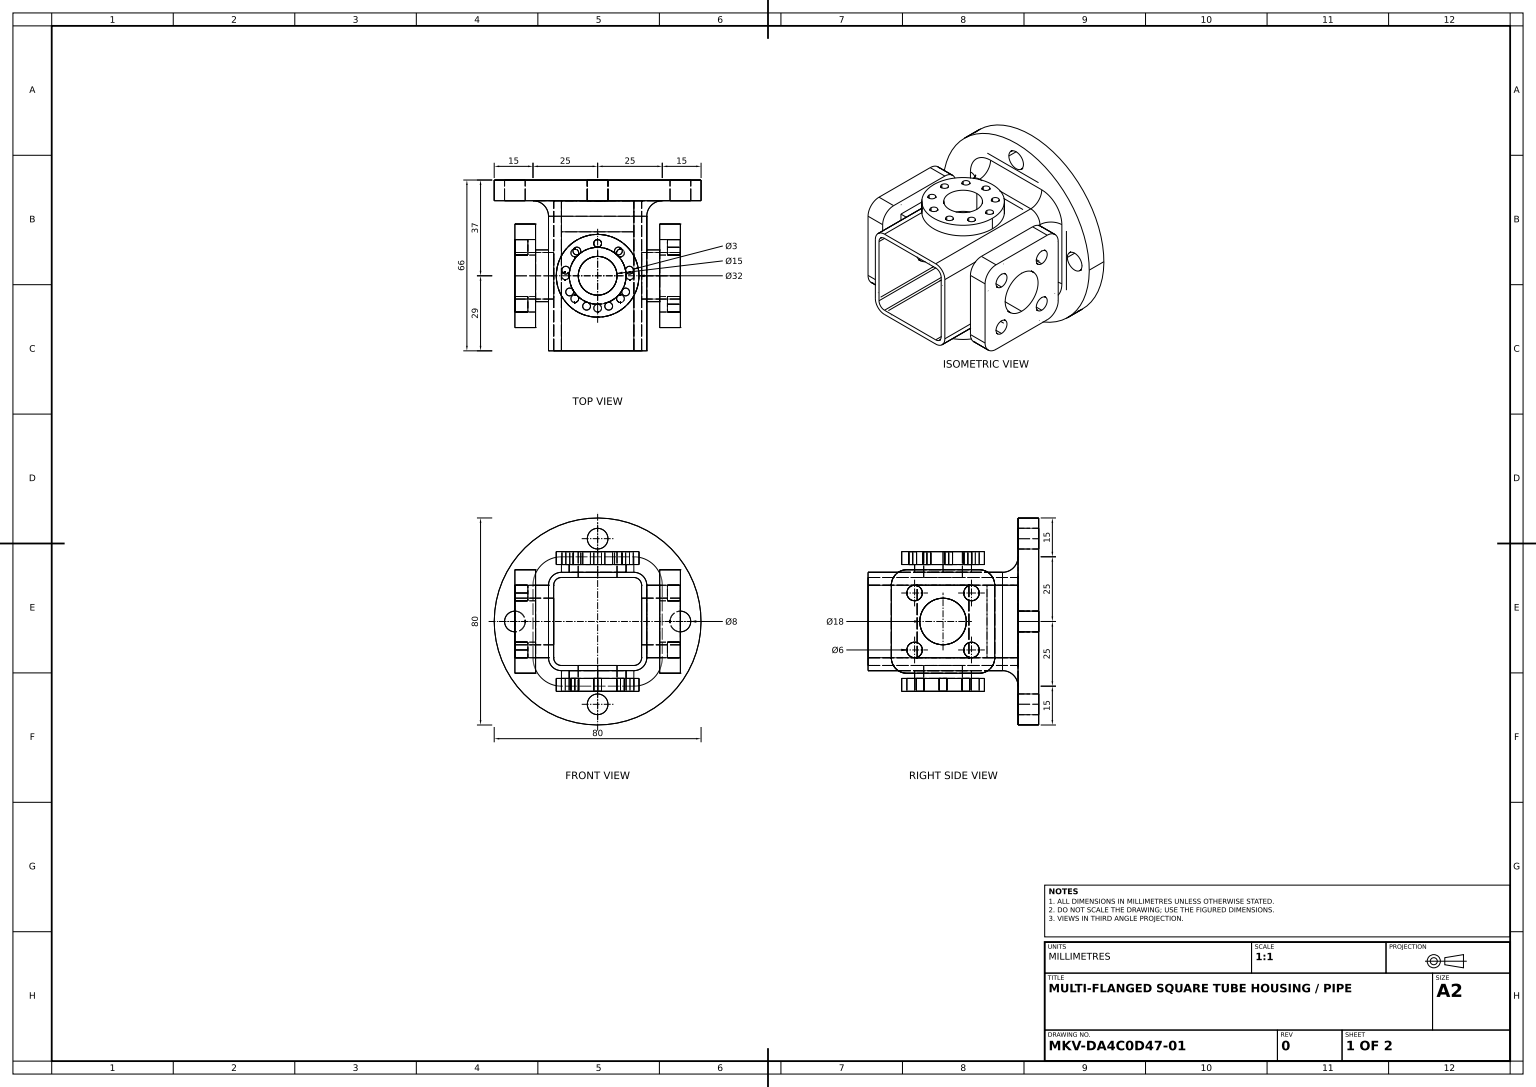
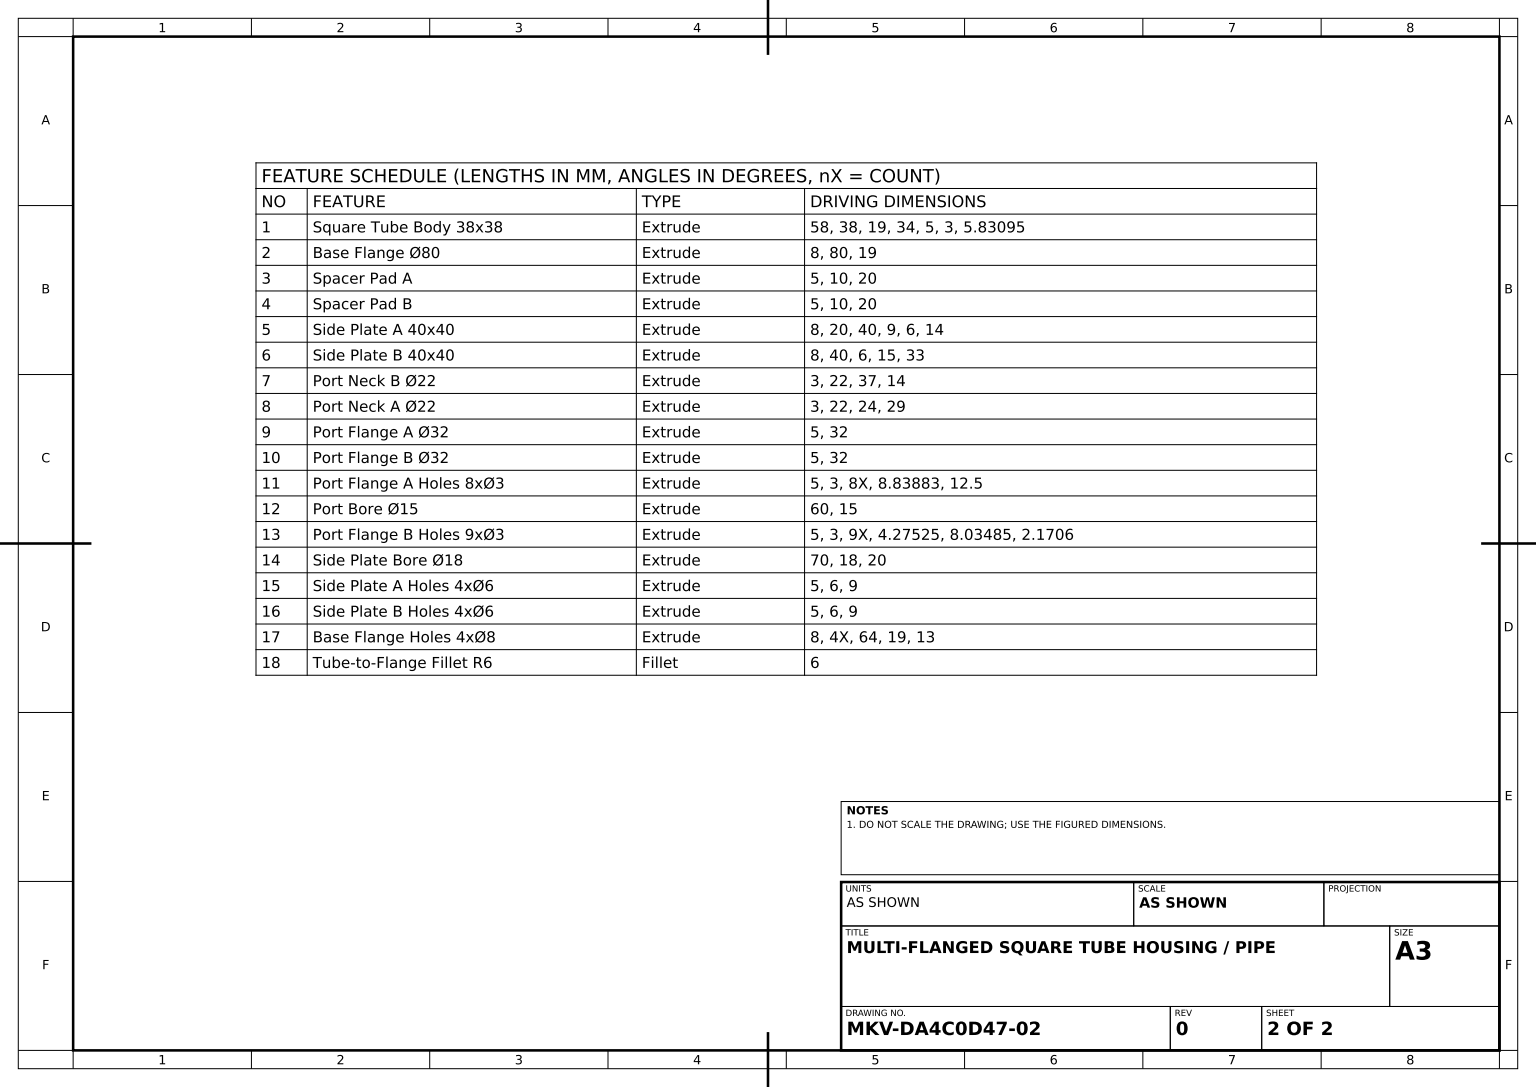
solid
v1 (-13,-33,9)
v2 (-5,-33,9)
e1 v1 v2 LINE
v3 (-13,-5,9)
e2 v3 v1 LINE
v4 (-5,-5,9)
e3 v3 v4 LINE
e4 v4 v2 LINE
face PLANE(AX(P(-13,-5,9),D(0,0,1),D(1,0,0))) rev [-e1 -e2 e3 e4]
v5 (6.674682,3,35.25)
v6 (6.674682,8,35.25)
e5 v5 v6 LINE
v7 (9.674682,8,35.25)
e6 v6 v7 CIRCLE(AX(P(8.174682,8,35.25),D(0,1,0),D(-1,0,0)),1.5)
v8 (9.674682,3,35.25)
e7 v8 v7 LINE
e8 v5 v8 CIRCLE(AX(P(8.174682,3,35.25),D(0,1,0),D(-1,0,0)),1.5)
face CYL(AX(P(8.174682,3,35.25),D(0,1,0),D(-1,0,0)),1.5) rev [e5 e6 -e7 -e8]
v9 (33,0,6)
v10 (33,6,0)
e9 v9 v10 CIRCLE(AX(P(33,6,6),D(1,0,0),D(0,1,0)),6)
v11 (38,-5,6)
e10 v11 v9 CIRCLE(AX(P(33,-5,6),D(0,0,1),D(-1,0,0)),5)
v12 (44,-5,0)
e11 v12 v11 CIRCLE(AX(P(44,-5,6),D(0,1,0),D(-1,0,0)),6)
e12 v10 v12 CIRCLE(AX(P(33,-5,0),D(0,0,-1),D(-1,0,0)),11)
face TORUS(AX(P(33,-5,6),D(0,0,-1),D(-1,0,0)),11,6) rev [-e9 -e10 -e11 -e12]
v13 (19,-41,13)
v14 (19,-41,45)
e13 v13 v14 CIRCLE(AX(P(19,-41,29),D(0,-1,0),D(0,0,-1)),16)
v15 (19,-46,45)
e14 v15 v14 LINE
v16 (19,-46,13)
e15 v16 v15 CIRCLE(AX(P(19,-46,29),D(0,-1,0),D(0,0,-1)),16)
e16 v16 v13 LINE
face CYL(AX(P(19,-46,29),D(0,1,0),D(0,0,1)),16) [e13 -e14 -e15 e16]
e17 v15 v16 CIRCLE(AX(P(19,-46,29),D(0,-1,0),D(0,0,-1)),16)
v17 (27.838835,-46,36.338835)
v18 (27.838835,-46,39.338835)
e18 v17 v18 CIRCLE(AX(P(27.838835,-46,37.838835),D(0,-1,0),D(0,0,-1)),1.5)
e19 v18 v17 CIRCLE(AX(P(27.838835,-46,37.838835),D(0,-1,0),D(0,0,-1)),1.5)
v19 (19,-46,40)
v20 (19,-46,43)
e20 v19 v20 CIRCLE(AX(P(19,-46,41.5),D(0,-1,0),D(0,0,-1)),1.5)
e21 v20 v19 CIRCLE(AX(P(19,-46,41.5),D(0,-1,0),D(0,0,-1)),1.5)
v21 (27.838835,-46,18.661165)
v22 (27.838835,-46,21.661165)
e22 v21 v22 CIRCLE(AX(P(27.838835,-46,20.161165),D(0,-1,0),D(0,0,-1)),1.5)
e23 v22 v21 CIRCLE(AX(P(27.838835,-46,20.161165),D(0,-1,0),D(0,0,-1)),1.5)
v23 (19,-46,21.5)
v24 (19,-46,36.5)
e24 v23 v24 CIRCLE(AX(P(19,-46,29),D(0,-1,0),D(0,0,-1)),7.5)
e25 v24 v23 CIRCLE(AX(P(19,-46,29),D(0,-1,0),D(0,0,-1)),7.5)
v25 (10.161165,-46,21.661165)
v26 (10.161165,-46,18.661165)
e26 v25 v26 CIRCLE(AX(P(10.161165,-46,20.161165),D(0,-1,0),D(0,0,-1)),1.5)
e27 v26 v25 CIRCLE(AX(P(10.161165,-46,20.161165),D(0,-1,0),D(0,0,-1)),1.5)
v27 (31.5,-46,30.5)
v28 (31.5,-46,27.5)
e28 v27 v28 CIRCLE(AX(P(31.5,-46,29),D(0,-1,0),D(0,0,-1)),1.5)
e29 v28 v27 CIRCLE(AX(P(31.5,-46,29),D(0,-1,0),D(0,0,-1)),1.5)
v29 (10.161165,-46,36.338835)
v30 (10.161165,-46,39.338835)
e30 v29 v30 CIRCLE(AX(P(10.161165,-46,37.838835),D(0,-1,0),D(0,0,-1)),1.5)
e31 v30 v29 CIRCLE(AX(P(10.161165,-46,37.838835),D(0,-1,0),D(0,0,-1)),1.5)
v31 (19,-46,15)
v32 (19,-46,18)
e32 v31 v32 CIRCLE(AX(P(19,-46,16.5),D(0,-1,0),D(0,0,-1)),1.5)
e33 v32 v31 CIRCLE(AX(P(19,-46,16.5),D(0,-1,0),D(0,0,-1)),1.5)
v33 (6.5,-46,30.5)
v34 (6.5,-46,27.5)
e34 v33 v34 CIRCLE(AX(P(6.5,-46,29),D(0,-1,0),D(0,0,-1)),1.5)
e35 v34 v33 CIRCLE(AX(P(6.5,-46,29),D(0,-1,0),D(0,0,-1)),1.5)
face PLANE(AX(P(19,-46,29),D(0,-1,0),D(0,0,-1))) [e15 e17] [-e18 -e19] [-e20 -e21] [-e22 -e23] [-e24 -e25] [-e26 -e27] [-e28 -e29] [-e30 -e31] [-e32 -e33] [-e34 -e35]
v35 (33,0,58)
e36 v35 v9 LINE
v36 (38,-5,58)
e37 v36 v35 CIRCLE(AX(P(33,-5,58),D(0,0,1),D(1,0,0)),5)
v37 (38,-5,39)
e38 v36 v37 LINE
v38 (38,-5,19)
e39 v38 v37 LINE
e40 v38 v11 LINE
face CYL(AX(P(33,-5,58),D(0,0,-1),D(-1,0,0)),5) [e10 -e36 -e37 e38 -e39 e40]
v39 (46,-11,18)
v40 (51,-11,18)
e41 v39 v40 LINE
v41 (46,-5,18)
e42 v41 v39 CIRCLE(AX(P(46,-8,18),D(1,0,0),D(0,1,0)),3)
v42 (51,-5,18)
e43 v41 v42 LINE
e44 v42 v40 CIRCLE(AX(P(51,-8,18),D(1,0,0),D(0,1,0)),3)
face CYL(AX(P(46,-8,18),D(1,0,0),D(0,1,0)),3) rev [-e41 -e42 e43 e44]
v43 (38,-33,39)
e45 v43 v37 LINE
v44 (43,-33,39)
e46 v44 v43 LINE
v45 (43,-5,39)
e47 v44 v45 LINE
e48 v45 v37 LINE
face PLANE(AX(P(43,0,39),D(0,0,1),D(0,-1,0))) [-e45 -e46 e47 e48]
v46 (-8,-8,43)
v47 (-8,-8,37)
e49 v46 v47 CIRCLE(AX(P(-8,-8,40),D(-1,0,0),D(0,0,1)),3)
e50 v47 v46 CIRCLE(AX(P(-8,-8,40),D(-1,0,0),D(0,0,1)),3)
face PLANE(AX(P(-8,-8,40),D(-1,0,0),D(0,0,1))) [e49 e50]
v48 (0,-33,6)
v49 (-6,-33,0)
e51 v48 v49 CIRCLE(AX(P(-6,-33,6),D(0,1,0),D(0,0,1)),6)
v50 (0,-5,6)
e52 v50 v48 LINE
v51 (-6,-5,0)
e53 v50 v51 CIRCLE(AX(P(-6,-5,6),D(0,1,0),D(-1,0,0)),6)
e54 v49 v51 LINE
face CYL(AX(P(-6,-33,6),D(0,1,0),D(0,0,1)),6) rev [-e51 -e52 e53 -e54]
v52 (5.189903,3,26.829398)
v53 (8.167115,3,27.08987)
e55 v52 v53 CIRCLE(AX(P(6.689903,3,26.829398),D(0,1,0),D(-1,0,0)),1.5)
v54 (8,3,29)
e56 v53 v54 CIRCLE(AX(P(19,3,29),D(0,1,0),D(-1,0,0)),11)
v55 (9.473721,3,34.5)
e57 v54 v55 CIRCLE(AX(P(19,3,29),D(0,1,0),D(-1,0,0)),11)
e58 v55 v5 CIRCLE(AX(P(8.174682,3,35.25),D(0,1,0),D(-1,0,0)),1.5)
e59 v8 v55 CIRCLE(AX(P(8.174682,3,35.25),D(0,1,0),D(-1,0,0)),1.5)
v56 (15.237778,3,39.336619)
e60 v55 v56 CIRCLE(AX(P(19,3,29),D(0,1,0),D(-1,0,0)),11)
v57 (13.224748,3,40.746158)
e61 v56 v57 CIRCLE(AX(P(14.724748,3,40.746158),D(0,1,0),D(-1,0,0)),1.5)
v58 (16.224748,3,40.746158)
e62 v57 v58 CIRCLE(AX(P(14.724748,3,40.746158),D(0,1,0),D(-1,0,0)),1.5)
e63 v58 v56 CIRCLE(AX(P(14.724748,3,40.746158),D(0,1,0),D(-1,0,0)),1.5)
v59 (22.762222,3,39.336619)
e64 v56 v59 CIRCLE(AX(P(19,3,29),D(0,1,0),D(-1,0,0)),11)
v60 (21.775252,3,40.746158)
e65 v59 v60 CIRCLE(AX(P(23.275252,3,40.746158),D(0,1,0),D(-1,0,0)),1.5)
v61 (24.775252,3,40.746158)
e66 v60 v61 CIRCLE(AX(P(23.275252,3,40.746158),D(0,1,0),D(-1,0,0)),1.5)
e67 v61 v59 CIRCLE(AX(P(23.275252,3,40.746158),D(0,1,0),D(-1,0,0)),1.5)
v62 (28.526279,3,34.5)
e68 v59 v62 CIRCLE(AX(P(19,3,29),D(0,1,0),D(-1,0,0)),11)
v63 (28.325318,3,35.25)
e69 v62 v63 CIRCLE(AX(P(29.825318,3,35.25),D(0,1,0),D(-1,0,0)),1.5)
v64 (31.325318,3,35.25)
e70 v63 v64 CIRCLE(AX(P(29.825318,3,35.25),D(0,1,0),D(-1,0,0)),1.5)
e71 v64 v62 CIRCLE(AX(P(29.825318,3,35.25),D(0,1,0),D(-1,0,0)),1.5)
v65 (30,3,29)
e72 v62 v65 CIRCLE(AX(P(19,3,29),D(0,1,0),D(-1,0,0)),11)
v66 (29.832885,3,27.08987)
e73 v65 v66 CIRCLE(AX(P(19,3,29),D(0,1,0),D(-1,0,0)),11)
v67 (32.810097,3,26.829398)
e74 v66 v67 CIRCLE(AX(P(31.310097,3,26.829398),D(0,1,0),D(-1,0,0)),1.5)
v68 (29.810097,3,26.829398)
e75 v67 v68 CIRCLE(AX(P(31.310097,3,26.829398),D(0,1,0),D(-1,0,0)),1.5)
e76 v68 v66 CIRCLE(AX(P(31.310097,3,26.829398),D(0,1,0),D(-1,0,0)),1.5)
v69 (26.070664,3,20.573511)
e77 v66 v69 CIRCLE(AX(P(19,3,29),D(0,1,0),D(-1,0,0)),11)
v70 (28.534845,3,19.424444)
e78 v69 v70 CIRCLE(AX(P(27.034845,3,19.424444),D(0,1,0),D(-1,0,0)),1.5)
v71 (25.534845,3,19.424444)
e79 v70 v71 CIRCLE(AX(P(27.034845,3,19.424444),D(0,1,0),D(-1,0,0)),1.5)
e80 v71 v69 CIRCLE(AX(P(27.034845,3,19.424444),D(0,1,0),D(-1,0,0)),1.5)
v72 (19,3,18)
e81 v69 v72 CIRCLE(AX(P(19,3,29),D(0,1,0),D(-1,0,0)),11)
v73 (20.5,3,16.5)
e82 v72 v73 CIRCLE(AX(P(19,3,16.5),D(0,1,0),D(-1,0,0)),1.5)
v74 (17.5,3,16.5)
e83 v73 v74 CIRCLE(AX(P(19,3,16.5),D(0,1,0),D(-1,0,0)),1.5)
e84 v74 v72 CIRCLE(AX(P(19,3,16.5),D(0,1,0),D(-1,0,0)),1.5)
v75 (11.929336,3,20.573511)
e85 v72 v75 CIRCLE(AX(P(19,3,29),D(0,1,0),D(-1,0,0)),11)
v76 (12.465155,3,19.424444)
e86 v75 v76 CIRCLE(AX(P(10.965155,3,19.424444),D(0,1,0),D(-1,0,0)),1.5)
v77 (9.465155,3,19.424444)
e87 v76 v77 CIRCLE(AX(P(10.965155,3,19.424444),D(0,1,0),D(-1,0,0)),1.5)
e88 v77 v75 CIRCLE(AX(P(10.965155,3,19.424444),D(0,1,0),D(-1,0,0)),1.5)
e89 v75 v53 CIRCLE(AX(P(19,3,29),D(0,1,0),D(-1,0,0)),11)
v78 (8.189903,3,26.829398)
e90 v53 v78 CIRCLE(AX(P(6.689903,3,26.829398),D(0,1,0),D(-1,0,0)),1.5)
e91 v78 v52 CIRCLE(AX(P(6.689903,3,26.829398),D(0,1,0),D(-1,0,0)),1.5)
v79 (3,3,29)
v80 (35,3,29)
e92 v79 v80 CIRCLE(AX(P(19,3,29),D(0,1,0),D(-1,0,0)),16)
e93 v80 v79 CIRCLE(AX(P(19,3,29),D(0,1,0),D(-1,0,0)),16)
face PLANE(AX(P(19,3,29),D(0,1,0),D(-1,0,0))) rev [e55 e56 e57 e58 e8 e59 e60 e61 e62 e63 e64 e65 e66 e67 e68 e69 e70 e71 e72 e73 e74 e75 e76 e77 e78 e79 e80 e81 e82 e83 e84 e85 e86 e87 e88 e89 e90 e91] [-e92 -e93]
v81 (15,-51,0)
v82 (15,-51,-8)
e94 v81 v82 LINE
v83 (23,-51,0)
e95 v83 v81 CIRCLE(AX(P(19,-51,0),D(0,0,-1),D(-1,0,0)),4)
v84 (23,-51,-8)
e96 v83 v84 LINE
e97 v84 v82 CIRCLE(AX(P(19,-51,-8),D(0,0,-1),D(-1,0,0)),4)
face CYL(AX(P(19,-51,0),D(0,0,-1),D(-1,0,0)),4) rev [-e94 -e95 e96 e97]
v85 (0,-33,58)
v86 (0,-33,39)
e98 v85 v86 LINE
v87 (0,-33,19)
e99 v87 v86 LINE
e100 v87 v48 LINE
v88 (5,-38,6)
e101 v48 v88 CIRCLE(AX(P(5,-33,6),D(0,0,1),D(-1,0,0)),5)
v89 (5,-38,58)
e102 v89 v88 LINE
e103 v85 v89 CIRCLE(AX(P(5,-33,58),D(0,0,1),D(-1,0,0)),5)
face CYL(AX(P(5,-33,58),D(0,0,-1),D(-1,0,0)),5) [e98 -e99 e100 e101 -e102 -e103]
v90 (33,-38,58)
v91 (38,-33,58)
e104 v90 v91 CIRCLE(AX(P(33,-33,58),D(0,0,1),D(1,0,0)),5)
e105 v91 v36 LINE
v92 (5,0,58)
e106 v35 v92 LINE
v93 (0,-5,58)
e107 v92 v93 CIRCLE(AX(P(5,-5,58),D(0,0,1),D(-1,0,0)),5)
e108 v93 v85 LINE
e109 v89 v90 LINE
v94 (36,-33,58)
v95 (36,-5,58)
e110 v94 v95 LINE
v96 (33,-36,58)
e111 v96 v94 CIRCLE(AX(P(33,-33,58),D(0,0,1),D(1,0,0)),3)
v97 (5,-36,58)
e112 v97 v96 LINE
v98 (2,-33,58)
e113 v98 v97 CIRCLE(AX(P(5,-33,58),D(0,0,1),D(-1,0,0)),3)
v99 (2,-5,58)
e114 v99 v98 LINE
v100 (5,-2,58)
e115 v100 v99 CIRCLE(AX(P(5,-5,58),D(0,0,1),D(1,0,0)),3)
v101 (33,-2,58)
e116 v101 v100 LINE
e117 v95 v101 CIRCLE(AX(P(33,-5,58),D(0,0,1),D(1,0,0)),3)
face PLANE(AX(P(5,-5,58),D(0,0,-1),D(-1,0,0))) rev [e104 e105 e37 e106 e107 e108 e103 e109] [-e110 -e111 -e112 -e113 -e114 -e115 -e116 -e117]
v102 (46,-33,40)
v103 (46,-27,40)
e118 v102 v103 CIRCLE(AX(P(46,-30,40),D(1,0,0),D(0,1,0)),3)
e119 v103 v102 CIRCLE(AX(P(46,-30,40),D(1,0,0),D(0,1,0)),3)
face PLANE(AX(P(46,-30,40),D(1,0,0),D(0,1,0))) [e118 e119]
v104 (36,-28,29)
v105 (36,-10,29)
e120 v104 v105 CIRCLE(AX(P(36,-19,29),D(-1,0,0),D(0,0,1)),9)
v106 (51,-10,29)
e121 v105 v106 LINE
v107 (51,-28,29)
e122 v106 v107 CIRCLE(AX(P(51,-19,29),D(1,0,0),D(0,1,0)),9)
e123 v104 v107 LINE
face CYL(AX(P(-19,-19,29),D(1,0,0),D(0,1,0)),9) rev [e120 e121 e122 -e123]
v108 (19,-41,18)
v109 (19,-41,15)
e124 v108 v109 CIRCLE(AX(P(19,-41,16.5),D(0,-1,0),D(0,0,-1)),1.5)
e125 v108 v32 LINE
e126 v109 v31 LINE
face CYL(AX(P(19,-41,16.5),D(0,-1,0),D(0,0,-1)),1.5) rev [-e124 e125 e33 -e126]
v110 (51,-33,9)
v111 (43,-33,9)
e127 v110 v111 LINE
v112 (43,-5,9)
e128 v111 v112 LINE
v113 (51,-5,9)
e129 v113 v112 LINE
e130 v110 v113 LINE
face PLANE(AX(P(51,-19,9),D(0,0,1),D(1,0,0))) rev [e127 e128 -e129 -e130]
v114 (31.5,-41,27.5)
e131 v114 v28 LINE
v115 (31.5,-41,30.5)
e132 v115 v27 LINE
e133 v114 v115 CIRCLE(AX(P(31.5,-41,29),D(0,-1,0),D(0,0,-1)),1.5)
face CYL(AX(P(31.5,-41,29),D(0,-1,0),D(0,0,-1)),1.5) rev [e131 e29 -e132 -e133]
v116 (10.161165,-41,21.661165)
e134 v116 v25 LINE
v117 (11.221825,-41,21.221825)
e135 v117 v116 CIRCLE(AX(P(10.161165,-41,20.161165),D(0,-1,0),D(0,0,-1)),1.5)
v118 (10.161165,-41,18.661165)
e136 v118 v117 CIRCLE(AX(P(10.161165,-41,20.161165),D(0,-1,0),D(0,0,-1)),1.5)
e137 v118 v26 LINE
face CYL(AX(P(10.161165,-41,20.161165),D(0,-1,0),D(0,0,-1)),1.5) rev [-e134 -e135 -e136 e137 e27]
v119 (51,-27,40)
e138 v103 v119 LINE
v120 (51,-33,40)
e139 v119 v120 CIRCLE(AX(P(51,-30,40),D(1,0,0),D(0,1,0)),3)
e140 v102 v120 LINE
face CYL(AX(P(46,-30,40),D(1,0,0),D(0,1,0)),3) rev [-e119 e138 e139 -e140]
v121 (32.810097,8,26.829398)
e141 v67 v121 LINE
v122 (29.810097,8,26.829398)
e142 v121 v122 CIRCLE(AX(P(31.310097,8,26.829398),D(0,1,0),D(-1,0,0)),1.5)
e143 v68 v122 LINE
face CYL(AX(P(31.310097,3,26.829398),D(0,1,0),D(-1,0,0)),1.5) rev [e141 e142 -e143 -e75]
v123 (19,-38,40)
v124 (19,-38,18)
e144 v123 v124 CIRCLE(AX(P(19,-38,29),D(0,-1,0),D(0,0,1)),11)
e145 v108 v124 LINE
e146 v117 v108 CIRCLE(AX(P(19,-41,29),D(0,-1,0),D(0,0,-1)),11)
v125 (8,-41,29)
e147 v125 v117 CIRCLE(AX(P(19,-41,29),D(0,-1,0),D(0,0,-1)),11)
v126 (11.221825,-41,36.778175)
e148 v126 v125 CIRCLE(AX(P(19,-41,29),D(0,-1,0),D(0,0,-1)),11)
v127 (19,-41,40)
e149 v127 v126 CIRCLE(AX(P(19,-41,29),D(0,-1,0),D(0,0,-1)),11)
e150 v127 v123 LINE
face CYL(AX(P(19,-41,29),D(0,1,0),D(0,0,1)),11) [e144 -e145 -e146 -e147 -e148 -e149 e150]
v128 (30,0,29)
v129 (8,0,29)
e151 v128 v129 CIRCLE(AX(P(19,0,29),D(0,1,0),D(1,0,0)),11)
e152 v129 v128 CIRCLE(AX(P(19,0,29),D(0,1,0),D(1,0,0)),11)
v130 (5,0,6)
e153 v92 v130 LINE
e154 v9 v130 LINE
face PLANE(AX(P(5,0,58),D(0,-1,0),D(1,0,0))) rev [-e151 -e152] [-e153 -e106 e36 e154]
v131 (-8,-30,15)
v132 (-8,-30,21)
e155 v131 v132 CIRCLE(AX(P(-8,-30,18),D(-1,0,0),D(0,0,1)),3)
v133 (-13,-30,15)
e156 v131 v133 LINE
v134 (-13,-30,21)
e157 v133 v134 CIRCLE(AX(P(-13,-30,18),D(-1,0,0),D(0,0,1)),3)
e158 v132 v134 LINE
face CYL(AX(P(-8,-30,18),D(-1,0,0),D(0,0,1)),3) rev [-e155 e156 e157 -e158]
e159 v7 v6 CIRCLE(AX(P(8.174682,8,35.25),D(0,1,0),D(-1,0,0)),1.5)
face CYL(AX(P(8.174682,3,35.25),D(0,1,0),D(-1,0,0)),1.5) rev [-e58 -e59 e7 e159 -e5]
v135 (15,13,-8)
v136 (23,13,-8)
e160 v135 v136 CIRCLE(AX(P(19,13,-8),D(0,0,-1),D(-1,0,0)),4)
v137 (23,13,0)
e161 v137 v136 LINE
v138 (15,13,0)
e162 v138 v137 CIRCLE(AX(P(19,13,0),D(0,0,-1),D(-1,0,0)),4)
e163 v138 v135 LINE
face CYL(AX(P(19,13,0),D(0,0,-1),D(-1,0,0)),4) rev [e160 -e161 -e162 e163]
e164 v136 v135 CIRCLE(AX(P(19,13,-8),D(0,0,-1),D(-1,0,0)),4)
e165 v137 v138 CIRCLE(AX(P(19,13,0),D(0,0,-1),D(-1,0,0)),4)
face CYL(AX(P(19,13,0),D(0,0,-1),D(-1,0,0)),4) rev [e164 -e163 -e165 e161]
v139 (2,-33,0)
v140 (5,-36,0)
e166 v139 v140 CIRCLE(AX(P(5,-33,0),D(0,0,1),D(-1,0,0)),3)
v141 (33,-36,0)
e167 v140 v141 LINE
v142 (36,-33,0)
e168 v141 v142 CIRCLE(AX(P(33,-33,0),D(0,0,1),D(1,0,0)),3)
v143 (36,-5,0)
e169 v142 v143 LINE
v144 (33,-2,0)
e170 v143 v144 CIRCLE(AX(P(33,-5,0),D(0,0,1),D(1,0,0)),3)
v145 (5,-2,0)
e171 v144 v145 LINE
v146 (2,-5,0)
e172 v145 v146 CIRCLE(AX(P(5,-5,0),D(0,0,1),D(1,0,0)),3)
e173 v146 v139 LINE
face PLANE(AX(P(19,-19,0),D(0,0,-1),D(-1,0,0))) rev [e166 e167 e168 e169 e170 e171 e172 e173]
v147 (-13,-39,15)
v148 (-13,-39,43)
e174 v147 v148 LINE
v149 (-5,-39,15)
e175 v147 v149 LINE
v150 (-5,-39,43)
e176 v149 v150 LINE
e177 v148 v150 LINE
face PLANE(AX(P(-13,-39,43),D(0,1,0),D(0,0,1))) rev [-e174 e175 e176 -e177]
v151 (19,-36,21.5)
e178 v151 v23 LINE
v152 (19,-36,36.5)
e179 v152 v24 LINE
e180 v152 v151 CIRCLE(AX(P(19,-36,29),D(0,1,0),D(0,0,1)),7.5)
face CYL(AX(P(19,14,29),D(0,-1,0),D(0,0,-1)),7.5) rev [e178 e24 -e179 e180]
v153 (28.534845,8,19.424444)
e181 v70 v153 LINE
v154 (25.534845,8,19.424444)
e182 v71 v154 LINE
e183 v154 v153 CIRCLE(AX(P(27.034845,8,19.424444),D(0,1,0),D(-1,0,0)),1.5)
face CYL(AX(P(27.034845,3,19.424444),D(0,1,0),D(-1,0,0)),1.5) rev [-e181 -e78 -e80 e182 e183]
v155 (-8,-30,43)
v156 (-8,-30,37)
e184 v155 v156 CIRCLE(AX(P(-8,-30,40),D(-1,0,0),D(0,0,1)),3)
v157 (-13,-30,43)
e185 v155 v157 LINE
v158 (-13,-30,37)
e186 v157 v158 CIRCLE(AX(P(-13,-30,40),D(-1,0,0),D(0,0,1)),3)
e187 v156 v158 LINE
face CYL(AX(P(-8,-30,40),D(-1,0,0),D(0,0,1)),3) rev [-e184 e185 e186 -e187]
v159 (13.224748,8,40.746158)
e188 v57 v159 LINE
v160 (16.224748,8,40.746158)
e189 v58 v160 LINE
e190 v160 v159 CIRCLE(AX(P(14.724748,8,40.746158),D(0,1,0),D(-1,0,0)),1.5)
face CYL(AX(P(14.724748,3,40.746158),D(0,1,0),D(-1,0,0)),1.5) rev [-e188 -e61 -e63 e189 e190]
v161 (-21,-19,-8)
v162 (-21,-19,0)
e191 v161 v162 LINE
v163 (59,-19,-8)
e192 v163 v161 CIRCLE(AX(P(19,-19,-8),D(0,0,-1),D(-1,0,0)),40)
v164 (59,-19,0)
e193 v163 v164 LINE
e194 v164 v162 CIRCLE(AX(P(19,-19,0),D(0,0,-1),D(-1,0,0)),40)
face CYL(AX(P(19,-19,-8),D(0,0,1),D(1,0,0)),40) [-e191 -e192 e193 e194]
v165 (8.189903,8,26.829398)
e195 v78 v165 LINE
v166 (5.189903,8,26.829398)
e196 v165 v166 CIRCLE(AX(P(6.689903,8,26.829398),D(0,1,0),D(-1,0,0)),1.5)
e197 v52 v166 LINE
face CYL(AX(P(6.689903,3,26.829398),D(0,1,0),D(-1,0,0)),1.5) rev [-e91 e195 e196 -e197]
e198 v132 v131 CIRCLE(AX(P(-8,-30,18),D(-1,0,0),D(0,0,1)),3)
e199 v134 v133 CIRCLE(AX(P(-13,-30,18),D(-1,0,0),D(0,0,1)),3)
face CYL(AX(P(-8,-30,18),D(-1,0,0),D(0,0,1)),3) rev [-e198 e158 e199 -e156]
e200 v81 v83 CIRCLE(AX(P(19,-51,0),D(0,0,-1),D(-1,0,0)),4)
e201 v82 v84 CIRCLE(AX(P(19,-51,-8),D(0,0,-1),D(-1,0,0)),4)
face CYL(AX(P(19,-51,0),D(0,0,-1),D(-1,0,0)),4) rev [-e96 -e200 e94 e201]
v167 (28.325318,8,35.25)
e202 v63 v167 LINE
v168 (31.325318,8,35.25)
e203 v64 v168 LINE
e204 v168 v167 CIRCLE(AX(P(29.825318,8,35.25),D(0,1,0),D(-1,0,0)),1.5)
face CYL(AX(P(29.825318,3,35.25),D(0,1,0),D(-1,0,0)),1.5) rev [-e202 -e69 -e71 e203 e204]
e205 v166 v165 CIRCLE(AX(P(6.689903,8,26.829398),D(0,1,0),D(-1,0,0)),1.5)
face CYL(AX(P(6.689903,3,26.829398),D(0,1,0),D(-1,0,0)),1.5) rev [-e195 -e90 -e55 e197 e205]
e206 v167 v168 CIRCLE(AX(P(29.825318,8,35.25),D(0,1,0),D(-1,0,0)),1.5)
face CYL(AX(P(29.825318,3,35.25),D(0,1,0),D(-1,0,0)),1.5) rev [e206 -e203 -e70 e202]
v169 (-5,-5,19)
v170 (0,-5,19)
e207 v169 v170 LINE
e208 v170 v87 LINE
v171 (-5,-33,19)
e209 v171 v87 LINE
e210 v169 v171 LINE
face PLANE(AX(P(-5,-33,19),D(0,0,1),D(0,-1,0))) rev [e207 e208 -e209 -e210]
v172 (24.775252,8,40.746158)
e211 v61 v172 LINE
v173 (21.775252,8,40.746158)
e212 v60 v173 LINE
e213 v173 v172 CIRCLE(AX(P(23.275252,8,40.746158),D(0,1,0),D(-1,0,0)),1.5)
face CYL(AX(P(23.275252,3,40.746158),D(0,1,0),D(-1,0,0)),1.5) rev [-e211 -e66 e212 e213]
v174 (38,-33,19)
e214 v43 v174 LINE
v175 (43,-33,19)
e215 v175 v174 LINE
e216 v44 v175 LINE
face PLANE(AX(P(43,-33,0),D(0,1,0),D(-1,0,0))) rev [e46 e214 -e215 -e216]
e217 v156 v155 CIRCLE(AX(P(-8,-30,40),D(-1,0,0),D(0,0,1)),3)
face PLANE(AX(P(-8,-30,40),D(-1,0,0),D(0,0,1))) [e184 e217]
v176 (33,-38,6)
v177 (38,-33,6)
e218 v176 v177 CIRCLE(AX(P(33,-33,6),D(0,0,1),D(-1,0,0)),5)
e219 v174 v177 LINE
e220 v91 v43 LINE
e221 v90 v176 LINE
face CYL(AX(P(33,-33,58),D(0,0,-1),D(-1,0,0)),5) [e218 -e219 -e214 -e220 -e104 e221]
v178 (-5,-5,39)
v179 (0,-5,39)
e222 v178 v179 LINE
e223 v179 v170 LINE
e224 v178 v169 LINE
face PLANE(AX(P(-5,-5,29),D(0,-1,0),D(0,0,-1))) rev [e222 e223 -e207 -e224]
v180 (47,-19,0)
v181 (47,-19,-8)
e225 v180 v181 LINE
v182 (55,-19,0)
e226 v182 v180 CIRCLE(AX(P(51,-19,0),D(0,0,-1),D(-1,0,0)),4)
v183 (55,-19,-8)
e227 v182 v183 LINE
e228 v183 v181 CIRCLE(AX(P(51,-19,-8),D(0,0,-1),D(-1,0,0)),4)
face CYL(AX(P(51,-19,0),D(0,0,-1),D(-1,0,0)),4) rev [-e225 -e226 e227 e228]
e229 v88 v176 LINE
e230 v124 v123 CIRCLE(AX(P(19,-38,29),D(0,-1,0),D(0,0,1)),11)
face PLANE(AX(P(33,-38,58),D(0,1,0),D(0,0,1))) rev [e102 e229 -e221 -e109] [-e144 -e230]
v184 (-5,-33,39)
e231 v171 v184 LINE
e232 v184 v178 LINE
e233 v2 v149 CIRCLE(AX(P(-5,-33,15),D(-1,0,0),D(0,0,-1)),6)
v185 (-5,1,15)
e234 v185 v4 CIRCLE(AX(P(-5,-5,15),D(-1,0,0),D(0,0,1)),6)
v186 (-5,1,43)
e235 v186 v185 LINE
v187 (-5,-5,49)
e236 v187 v186 CIRCLE(AX(P(-5,-5,43),D(-1,0,0),D(0,0,1)),6)
v188 (-5,-33,49)
e237 v188 v187 LINE
e238 v150 v188 CIRCLE(AX(P(-5,-33,43),D(-1,0,0),D(0,0,1)),6)
face PLANE(AX(P(-5,-33,15),D(1,0,0),D(0,0,-1))) [e224 e210 e231 e232] [-e233 -e4 -e234 -e235 -e236 -e237 -e238 -e176]
e239 v162 v164 CIRCLE(AX(P(19,-19,0),D(0,0,-1),D(-1,0,0)),40)
e240 v161 v163 CIRCLE(AX(P(19,-19,-8),D(0,0,-1),D(-1,0,0)),40)
face CYL(AX(P(19,-19,-8),D(0,0,1),D(1,0,0)),40) [e191 e239 -e193 -e240]
v189 (19,8,21.5)
v190 (19,-2,21.5)
e241 v189 v190 LINE
v191 (19,-2,36.5)
e242 v190 v191 CIRCLE(AX(P(19,-2,29),D(0,-1,0),D(0,0,-1)),7.5)
v192 (19,8,36.5)
e243 v192 v191 LINE
e244 v192 v189 CIRCLE(AX(P(19,8,29),D(0,1,0),D(-1,0,0)),7.5)
face CYL(AX(P(19,14,29),D(0,-1,0),D(0,0,-1)),7.5) rev [e241 e242 -e243 e244]
v193 (5,6,0)
e245 v193 v10 LINE
e246 v130 v193 CIRCLE(AX(P(5,6,6),D(1,0,0),D(0,0,-1)),6)
face CYL(AX(P(5,6,6),D(1,0,0),D(0,1,0)),6) rev [-e245 -e246 -e154 e9]
v194 (35,8,29)
v195 (3,8,29)
e247 v194 v195 CIRCLE(AX(P(19,8,29),D(0,1,0),D(-1,0,0)),16)
e248 v194 v80 LINE
e249 v195 v79 LINE
face CYL(AX(P(19,8,29),D(0,-1,0),D(1,0,0)),16) [-e247 e248 e93 -e249]
v196 (-13,-33,49)
e250 v196 v188 LINE
e251 v148 v196 CIRCLE(AX(P(-13,-33,43),D(-1,0,0),D(0,0,1)),6)
face CYL(AX(P(-13,-33,43),D(1,0,0),D(0,0,-1)),6) [e177 e238 -e250 -e251]
v197 (9.465155,8,19.424444)
e252 v77 v197 LINE
v198 (12.465155,8,19.424444)
e253 v76 v198 LINE
e254 v198 v197 CIRCLE(AX(P(10.965155,8,19.424444),D(0,1,0),D(-1,0,0)),1.5)
face CYL(AX(P(10.965155,3,19.424444),D(0,1,0),D(-1,0,0)),1.5) rev [-e252 -e87 e253 e254]
v199 (30,-41,29)
e255 v115 v199 CIRCLE(AX(P(31.5,-41,29),D(0,-1,0),D(0,0,-1)),1.5)
e256 v199 v114 CIRCLE(AX(P(31.5,-41,29),D(0,-1,0),D(0,0,-1)),1.5)
face CYL(AX(P(31.5,-41,29),D(0,-1,0),D(0,0,-1)),1.5) rev [-e255 e132 e28 -e131 -e256]
v200 (46,-5,40)
v201 (46,-11,40)
e257 v200 v201 CIRCLE(AX(P(46,-8,40),D(1,0,0),D(0,1,0)),3)
e258 v201 v200 CIRCLE(AX(P(46,-8,40),D(1,0,0),D(0,1,0)),3)
face PLANE(AX(P(46,-8,40),D(1,0,0),D(0,1,0))) [e257 e258]
e259 v184 v86 LINE
face PLANE(AX(P(-5,-33,39),D(0,1,0),D(0,0,1))) rev [-e231 e209 e99 -e259]
e260 v86 v179 LINE
e261 v93 v179 LINE
face PLANE(AX(P(0,-33,58),D(1,0,0),D(0,0,-1))) rev [-e260 -e98 -e108 e261]
v202 (-13,1,43)
e262 v202 v186 LINE
v203 (-13,-5,49)
e263 v203 v202 CIRCLE(AX(P(-13,-5,43),D(-1,0,0),D(0,0,1)),6)
e264 v203 v187 LINE
face CYL(AX(P(-13,-5,43),D(1,0,0),D(0,0,-1)),6) [e236 -e262 -e263 e264]
e265 v170 v50 LINE
face PLANE(AX(P(0,-33,58),D(1,0,0),D(0,0,-1))) rev [e265 e52 -e100 -e208]
v204 (27.838835,-41,36.338835)
e266 v204 v17 LINE
v205 (26.778175,-41,36.778175)
e267 v205 v204 CIRCLE(AX(P(27.838835,-41,37.838835),D(0,-1,0),D(0,0,-1)),1.5)
v206 (27.838835,-41,39.338835)
e268 v206 v205 CIRCLE(AX(P(27.838835,-41,37.838835),D(0,-1,0),D(0,0,-1)),1.5)
e269 v206 v18 LINE
face CYL(AX(P(27.838835,-41,37.838835),D(0,-1,0),D(0,0,-1)),1.5) rev [e19 -e266 -e267 -e268 e269]
e270 v197 v198 CIRCLE(AX(P(10.965155,8,19.424444),D(0,1,0),D(-1,0,0)),1.5)
face CYL(AX(P(10.965155,3,19.424444),D(0,1,0),D(-1,0,0)),1.5) rev [-e253 -e86 -e88 e252 e270]
e271 v65 v128 LINE
e272 v54 v129 LINE
face CYL(AX(P(19,3,29),D(0,-1,0),D(1,0,0)),11) [-e77 -e73 e271 e151 -e272 -e56 -e89 -e85 -e81]
e273 v177 v11 LINE
e274 v38 v174 LINE
face PLANE(AX(P(38,-5,58),D(-1,0,0),D(0,-1,0))) rev [e219 e273 -e40 e274]
e275 v51 v193 CIRCLE(AX(P(5,-5,0),D(0,0,-1),D(-1,0,0)),11)
e276 v130 v50 CIRCLE(AX(P(5,-5,6),D(0,0,1),D(-1,0,0)),5)
face TORUS(AX(P(5,-5,6),D(0,0,-1),D(-1,0,0)),11,6) rev [e246 -e275 -e53 -e276]
e277 v98 v139 LINE
e278 v97 v140 LINE
face CYL(AX(P(5,-33,58),D(0,0,-1),D(-1,0,0)),3) rev [-e166 -e277 e113 e278]
v207 (5,-44,0)
e279 v207 v88 CIRCLE(AX(P(5,-44,6),D(1,0,0),D(0,1,0)),6)
e280 v207 v49 CIRCLE(AX(P(5,-33,0),D(0,0,-1),D(-1,0,0)),11)
face TORUS(AX(P(5,-33,6),D(0,0,-1),D(-1,0,0)),11,6) rev [e279 -e101 e51 -e280]
e281 v127 v19 LINE
v208 (19,-41,43)
e282 v208 v127 CIRCLE(AX(P(19,-41,41.5),D(0,-1,0),D(0,0,-1)),1.5)
e283 v208 v20 LINE
face CYL(AX(P(19,-41,41.5),D(0,-1,0),D(0,0,-1)),1.5) rev [e21 -e281 -e282 e283]
v209 (43,-33,49)
v210 (43,-39,43)
e284 v209 v210 CIRCLE(AX(P(43,-33,43),D(1,0,0),D(0,-1,0)),6)
v211 (51,-39,43)
e285 v211 v210 LINE
v212 (51,-33,49)
e286 v212 v211 CIRCLE(AX(P(51,-33,43),D(1,0,0),D(0,-1,0)),6)
e287 v212 v209 LINE
face CYL(AX(P(51,-33,43),D(-1,0,0),D(0,-1,0)),6) [e284 -e285 -e286 e287]
e288 v191 v190 CIRCLE(AX(P(19,-2,29),D(0,-1,0),D(0,0,-1)),7.5)
e289 v189 v192 CIRCLE(AX(P(19,8,29),D(0,1,0),D(-1,0,0)),7.5)
face CYL(AX(P(19,14,29),D(0,-1,0),D(0,0,-1)),7.5) rev [e243 e288 -e241 e289]
e290 v39 v41 CIRCLE(AX(P(46,-8,18),D(1,0,0),D(0,1,0)),3)
face PLANE(AX(P(46,-8,18),D(1,0,0),D(0,1,0))) [e290 e42]
v213 (51,1,15)
e291 v113 v213 CIRCLE(AX(P(51,-5,15),D(1,0,0),D(0,1,0)),6)
v214 (43,1,15)
e292 v112 v214 CIRCLE(AX(P(43,-5,15),D(1,0,0),D(0,1,0)),6)
e293 v213 v214 LINE
face CYL(AX(P(51,-5,15),D(-1,0,0),D(0,-1,0)),6) [-e291 e129 e292 -e293]
v215 (-13,-10,29)
v216 (-13,-28,29)
e294 v215 v216 CIRCLE(AX(P(-13,-19,29),D(1,0,0),D(0,0,-1)),9)
e295 v216 v215 CIRCLE(AX(P(-13,-19,29),D(1,0,0),D(0,0,-1)),9)
v217 (-13,-8,43)
v218 (-13,-8,37)
e296 v217 v218 CIRCLE(AX(P(-13,-8,40),D(-1,0,0),D(0,0,1)),3)
e297 v218 v217 CIRCLE(AX(P(-13,-8,40),D(-1,0,0),D(0,0,1)),3)
v219 (-13,-8,15)
v220 (-13,-8,21)
e298 v219 v220 CIRCLE(AX(P(-13,-8,18),D(-1,0,0),D(0,0,1)),3)
e299 v220 v219 CIRCLE(AX(P(-13,-8,18),D(-1,0,0),D(0,0,1)),3)
e300 v158 v157 CIRCLE(AX(P(-13,-30,40),D(-1,0,0),D(0,0,1)),3)
e301 v1 v147 CIRCLE(AX(P(-13,-33,15),D(-1,0,0),D(0,0,-1)),6)
e302 v196 v203 LINE
v221 (-13,1,15)
e303 v202 v221 LINE
e304 v221 v3 CIRCLE(AX(P(-13,-5,15),D(-1,0,0),D(0,0,1)),6)
face PLANE(AX(P(-13,-33,15),D(1,0,0),D(0,0,-1))) rev [e294 e295] [-e296 -e297] [-e298 -e299] [-e157 -e199] [-e300 -e186] [e2 e301 e174 e251 e302 e263 e303 e304]
e305 v40 v42 CIRCLE(AX(P(51,-8,18),D(1,0,0),D(0,1,0)),3)
face CYL(AX(P(46,-8,18),D(1,0,0),D(0,1,0)),3) rev [e305 -e43 -e290 e41]
e306 v109 v108 CIRCLE(AX(P(19,-41,16.5),D(0,-1,0),D(0,0,-1)),1.5)
face CYL(AX(P(19,-41,16.5),D(0,-1,0),D(0,0,-1)),1.5) rev [-e125 -e306 e126 e32]
e307 v101 v144 LINE
e308 v100 v145 LINE
face PLANE(AX(P(5,-2,58),D(0,-1,0),D(0,0,-1))) [-e288 -e242] [-e171 -e307 e116 e308]
e309 v151 v152 CIRCLE(AX(P(19,-36,29),D(0,1,0),D(0,0,1)),7.5)
face CYL(AX(P(19,14,29),D(0,-1,0),D(0,0,-1)),7.5) rev [e179 e25 -e178 e309]
e310 v204 v206 CIRCLE(AX(P(27.838835,-41,37.838835),D(0,-1,0),D(0,0,-1)),1.5)
face CYL(AX(P(27.838835,-41,37.838835),D(0,-1,0),D(0,0,-1)),1.5) rev [-e269 -e310 e266 e18]
face CYL(AX(P(19,3,29),D(0,-1,0),D(1,0,0)),11) [-e60 -e57 e272 e152 -e271 -e72 -e68 -e64]
v222 (6.5,-41,30.5)
e311 v222 v33 LINE
e312 v125 v222 CIRCLE(AX(P(6.5,-41,29),D(0,-1,0),D(0,0,-1)),1.5)
v223 (6.5,-41,27.5)
e313 v223 v125 CIRCLE(AX(P(6.5,-41,29),D(0,-1,0),D(0,0,-1)),1.5)
e314 v223 v34 LINE
face CYL(AX(P(6.5,-41,29),D(0,-1,0),D(0,0,-1)),1.5) rev [-e311 -e312 -e313 e314 e35]
v224 (43,-5,19)
e315 v224 v38 LINE
e316 v224 v175 LINE
face PLANE(AX(P(43,0,19),D(0,0,-1),D(0,1,0))) [e215 -e274 -e315 e316]
e317 v46 v217 LINE
e318 v47 v218 LINE
face CYL(AX(P(-8,-8,40),D(-1,0,0),D(0,0,1)),3) rev [e297 -e317 -e50 e318]
v225 (51,-11,40)
v226 (51,-5,40)
e319 v225 v226 CIRCLE(AX(P(51,-8,40),D(1,0,0),D(0,1,0)),3)
e320 v226 v225 CIRCLE(AX(P(51,-8,40),D(1,0,0),D(0,1,0)),3)
v227 (51,1,43)
e321 v213 v227 LINE
v228 (51,-5,49)
e322 v227 v228 CIRCLE(AX(P(51,-5,43),D(1,0,0),D(0,1,0)),6)
e323 v228 v212 LINE
v229 (51,-39,15)
e324 v211 v229 LINE
e325 v229 v110 CIRCLE(AX(P(51,-33,15),D(1,0,0),D(0,1,0)),6)
v230 (51,-33,18)
v231 (51,-27,18)
e326 v230 v231 CIRCLE(AX(P(51,-30,18),D(1,0,0),D(0,1,0)),3)
e327 v231 v230 CIRCLE(AX(P(51,-30,18),D(1,0,0),D(0,1,0)),3)
e328 v120 v119 CIRCLE(AX(P(51,-30,40),D(1,0,0),D(0,1,0)),3)
e329 v107 v106 CIRCLE(AX(P(51,-19,29),D(1,0,0),D(0,1,0)),9)
face PLANE(AX(P(51,-5,15),D(1,0,0),D(0,1,0))) [-e44 -e305] [-e319 -e320] [e321 e322 e323 e286 e324 e325 e130 e291] [-e326 -e327] [-e139 -e328] [-e329 -e122]
e330 v96 v141 LINE
face PLANE(AX(P(33,-36,58),D(0,1,0),D(0,0,1))) [-e167 -e278 e112 e330] [-e309 -e180]
v232 (46,-33,18)
v233 (46,-27,18)
e331 v232 v233 CIRCLE(AX(P(46,-30,18),D(1,0,0),D(0,1,0)),3)
e332 v233 v232 CIRCLE(AX(P(46,-30,18),D(1,0,0),D(0,1,0)),3)
face PLANE(AX(P(46,-30,18),D(1,0,0),D(0,1,0))) [e331 e332]
e333 v153 v154 CIRCLE(AX(P(27.034845,8,19.424444),D(0,1,0),D(-1,0,0)),1.5)
face CYL(AX(P(27.034845,3,19.424444),D(0,1,0),D(-1,0,0)),1.5) rev [-e79 e181 e333 -e182]
v234 (-8,-8,21)
v235 (-8,-8,15)
e334 v234 v235 CIRCLE(AX(P(-8,-8,18),D(-1,0,0),D(0,0,1)),3)
e335 v235 v234 CIRCLE(AX(P(-8,-8,18),D(-1,0,0),D(0,0,1)),3)
face PLANE(AX(P(-8,-8,18),D(-1,0,0),D(0,0,1))) [e334 e335]
v236 (-17,-19,-8)
v237 (-9,-19,-8)
e336 v236 v237 CIRCLE(AX(P(-13,-19,-8),D(0,0,-1),D(-1,0,0)),4)
v238 (-9,-19,0)
e337 v238 v237 LINE
v239 (-17,-19,0)
e338 v239 v238 CIRCLE(AX(P(-13,-19,0),D(0,0,-1),D(-1,0,0)),4)
e339 v239 v236 LINE
face CYL(AX(P(-13,-19,0),D(0,0,-1),D(-1,0,0)),4) rev [e336 -e337 -e338 e339]
face CYL(AX(P(-8,-8,40),D(-1,0,0),D(0,0,1)),3) rev [e296 -e318 -e49 e317]
face PLANE(AX(P(-5,-5,39),D(0,0,-1),D(0,1,0))) rev [-e232 e259 e260 -e222]
v240 (43,-5,49)
e340 v228 v240 LINE
v241 (43,1,43)
e341 v227 v241 LINE
e342 v241 v240 CIRCLE(AX(P(43,-5,43),D(1,0,0),D(0,1,0)),6)
face CYL(AX(P(51,-5,43),D(-1,0,0),D(0,-1,0)),6) [-e340 -e322 e341 e342]
e343 v224 v45 LINE
v242 (43,-39,15)
e344 v210 v242 LINE
e345 v240 v209 LINE
e346 v214 v241 LINE
e347 v242 v111 CIRCLE(AX(P(43,-33,15),D(1,0,0),D(0,1,0)),6)
face PLANE(AX(P(43,-5,15),D(1,0,0),D(0,1,0))) rev [e343 -e47 e216 -e316] [-e344 -e284 -e345 -e342 -e346 -e292 -e128 -e347]
face CYL(AX(P(5,-5,58),D(0,0,-1),D(-1,0,0)),5) [-e107 e153 e276 -e265 -e223 -e261]
face PLANE(AX(P(51,-5,49),D(0,0,-1),D(-1,0,0))) rev [e345 -e287 -e323 e340]
face CYL(AX(P(-13,-33,15),D(1,0,0),D(0,0,-1)),6) [-e301 e1 e233 -e175]
v243 (26.778175,-41,21.221825)
v244 (27.838835,-41,18.661165)
e348 v243 v244 CIRCLE(AX(P(27.838835,-41,20.161165),D(0,-1,0),D(0,0,-1)),1.5)
v245 (27.838835,-41,21.661165)
e349 v244 v245 CIRCLE(AX(P(27.838835,-41,20.161165),D(0,-1,0),D(0,0,-1)),1.5)
e350 v245 v243 CIRCLE(AX(P(27.838835,-41,20.161165),D(0,-1,0),D(0,0,-1)),1.5)
e351 v243 v199 CIRCLE(AX(P(19,-41,29),D(0,-1,0),D(0,0,-1)),11)
e352 v199 v205 CIRCLE(AX(P(19,-41,29),D(0,-1,0),D(0,0,-1)),11)
e353 v205 v127 CIRCLE(AX(P(19,-41,29),D(0,-1,0),D(0,0,-1)),11)
e354 v127 v208 CIRCLE(AX(P(19,-41,41.5),D(0,-1,0),D(0,0,-1)),1.5)
v246 (10.161165,-41,39.338835)
e355 v126 v246 CIRCLE(AX(P(10.161165,-41,37.838835),D(0,-1,0),D(0,0,-1)),1.5)
v247 (10.161165,-41,36.338835)
e356 v246 v247 CIRCLE(AX(P(10.161165,-41,37.838835),D(0,-1,0),D(0,0,-1)),1.5)
e357 v247 v126 CIRCLE(AX(P(10.161165,-41,37.838835),D(0,-1,0),D(0,0,-1)),1.5)
e358 v222 v223 CIRCLE(AX(P(6.5,-41,29),D(0,-1,0),D(0,0,-1)),1.5)
e359 v116 v118 CIRCLE(AX(P(10.161165,-41,20.161165),D(0,-1,0),D(0,0,-1)),1.5)
e360 v108 v243 CIRCLE(AX(P(19,-41,29),D(0,-1,0),D(0,0,-1)),11)
e361 v14 v13 CIRCLE(AX(P(19,-41,29),D(0,-1,0),D(0,0,-1)),16)
face PLANE(AX(P(19,-41,29),D(0,-1,0),D(0,0,-1))) rev [e348 e349 e350 e351 e256 e133 e255 e352 e267 e310 e268 e353 e354 e282 e149 e355 e356 e357 e148 e312 e358 e313 e147 e135 e359 e136 e146 e124 e306 e360] [-e361 -e13]
v248 (33,-44,0)
e362 v248 v207 LINE
e363 v248 v176 CIRCLE(AX(P(33,-44,6),D(1,0,0),D(0,1,0)),6)
face CYL(AX(P(33,-44,6),D(-1,0,0),D(0,0,1)),6) rev [-e229 -e279 -e362 e363]
e364 v246 v30 LINE
e365 v247 v29 LINE
face CYL(AX(P(10.161165,-41,37.838835),D(0,-1,0),D(0,0,-1)),1.5) rev [-e356 e364 e31 -e365]
e366 v237 v236 CIRCLE(AX(P(-13,-19,-8),D(0,0,-1),D(-1,0,0)),4)
e367 v238 v239 CIRCLE(AX(P(-13,-19,0),D(0,0,-1),D(-1,0,0)),4)
face CYL(AX(P(-13,-19,0),D(0,0,-1),D(-1,0,0)),4) rev [e337 e366 -e339 -e367]
e368 v229 v242 LINE
face PLANE(AX(P(51,-39,43),D(0,1,0),D(-1,0,0))) rev [-e324 e285 e344 -e368]
face CYL(AX(P(46,-30,40),D(1,0,0),D(0,1,0)),3) rev [e328 -e138 -e118 e140]
v249 (2,-28,29)
e369 v216 v249 LINE
v250 (2,-10,29)
e370 v249 v250 CIRCLE(AX(P(2,-19,29),D(1,0,0),D(0,0,-1)),9)
e371 v215 v250 LINE
face CYL(AX(P(-19,-19,29),D(1,0,0),D(0,1,0)),9) rev [-e295 e369 e370 -e371]
e372 v234 v220 LINE
e373 v235 v219 LINE
face CYL(AX(P(-8,-8,18),D(-1,0,0),D(0,0,1)),3) rev [e298 -e372 -e335 e373]
e374 v244 v21 LINE
e375 v245 v22 LINE
face CYL(AX(P(27.838835,-41,20.161165),D(0,-1,0),D(0,0,-1)),1.5) rev [-e349 e374 e22 -e375]
v251 (44,-33,0)
e376 v251 v248 CIRCLE(AX(P(33,-33,0),D(0,0,-1),D(-1,0,0)),11)
e377 v251 v177 CIRCLE(AX(P(44,-33,6),D(0,1,0),D(0,0,1)),6)
face TORUS(AX(P(33,-33,6),D(0,0,-1),D(-1,0,0)),11,6) rev [-e376 e377 -e218 -e363]
face CYL(AX(P(10.161165,-41,20.161165),D(0,-1,0),D(0,0,-1)),1.5) rev [-e137 -e359 e134 e26]
face CYL(AX(P(10.161165,-41,37.838835),D(0,-1,0),D(0,0,-1)),1.5) rev [-e364 -e355 -e357 e365 e30]
e378 v180 v182 CIRCLE(AX(P(51,-19,0),D(0,0,-1),D(-1,0,0)),4)
e379 v181 v183 CIRCLE(AX(P(51,-19,-8),D(0,0,-1),D(-1,0,0)),4)
face CYL(AX(P(51,-19,0),D(0,0,-1),D(-1,0,0)),4) rev [-e378 e225 e379 -e227]
face PLANE(AX(P(19,-19,-8),D(0,0,-1),D(-1,0,0))) [-e366 -e336] [-e160 -e164] [-e379 -e228] [e192 e240] [-e201 -e97]
face PLANE(AX(P(43,-5,0),D(0,-1,0),D(1,0,0))) rev [e315 e39 -e48 -e343]
v252 (17.5,8,16.5)
e380 v74 v252 LINE
v253 (20.5,8,16.5)
e381 v73 v253 LINE
e382 v253 v252 CIRCLE(AX(P(19,8,16.5),D(0,1,0),D(-1,0,0)),1.5)
face CYL(AX(P(19,3,16.5),D(0,1,0),D(-1,0,0)),1.5) rev [-e380 -e83 e381 e382]
face PLANE(AX(P(-13,-5,49),D(0,0,-1),D(-1,0,0))) rev [-e302 e250 e237 -e264]
e383 v159 v160 CIRCLE(AX(P(14.724748,8,40.746158),D(0,1,0),D(-1,0,0)),1.5)
face CYL(AX(P(14.724748,3,40.746158),D(0,1,0),D(-1,0,0)),1.5) rev [e383 -e189 -e62 e188]
face PLANE(AX(P(-8,-30,18),D(-1,0,0),D(0,0,1))) [e155 e198]
e384 v12 v251 LINE
face CYL(AX(P(44,-5,6),D(0,-1,0),D(1,0,0)),6) rev [-e273 -e377 -e384 e11]
e385 v94 v142 LINE
face CYL(AX(P(33,-33,58),D(0,0,-1),D(-1,0,0)),3) rev [e111 e385 -e168 -e330]
e386 v221 v185 LINE
face PLANE(AX(P(-13,1,15),D(0,-1,0),D(0,0,-1))) rev [-e303 e262 e235 -e386]
face CYL(AX(P(-13,-5,15),D(1,0,0),D(0,0,-1)),6) [e234 -e3 -e304 e386]
e387 v195 v194 CIRCLE(AX(P(19,8,29),D(0,1,0),D(-1,0,0)),16)
e388 v172 v173 CIRCLE(AX(P(23.275252,8,40.746158),D(0,1,0),D(-1,0,0)),1.5)
e389 v252 v253 CIRCLE(AX(P(19,8,16.5),D(0,1,0),D(-1,0,0)),1.5)
e390 v122 v121 CIRCLE(AX(P(31.310097,8,26.829398),D(0,1,0),D(-1,0,0)),1.5)
face PLANE(AX(P(19,8,29),D(0,1,0),D(-1,0,0))) [e247 e387] [-e204 -e206] [-e333 -e183] [-e159 -e6] [-e190 -e383] [-e205 -e196] [-e270 -e254] [-e213 -e388] [-e389 -e382] [-e390 -e142] [-e289 -e244]
e391 v200 v226 LINE
e392 v201 v225 LINE
face CYL(AX(P(46,-8,40),D(1,0,0),D(0,1,0)),3) rev [-e257 e391 e320 -e392]
face CYL(AX(P(-8,-8,18),D(-1,0,0),D(0,0,1)),3) rev [-e334 e372 e299 -e373]
face CYL(AX(P(19,3,16.5),D(0,1,0),D(-1,0,0)),1.5) rev [e389 -e381 -e82 -e84 e380]
e393 v250 v249 CIRCLE(AX(P(2,-19,29),D(1,0,0),D(0,0,-1)),9)
face CYL(AX(P(-19,-19,29),D(1,0,0),D(0,1,0)),9) rev [-e294 e371 e393 -e369]
e394 v105 v104 CIRCLE(AX(P(36,-19,29),D(-1,0,0),D(0,0,1)),9)
face CYL(AX(P(-19,-19,29),D(1,0,0),D(0,1,0)),9) rev [-e121 e394 e123 e329]
e395 v233 v231 LINE
e396 v232 v230 LINE
face CYL(AX(P(46,-30,18),D(1,0,0),D(0,1,0)),3) rev [-e395 -e331 e396 e326]
face CYL(AX(P(46,-8,40),D(1,0,0),D(0,1,0)),3) rev [e319 -e391 -e258 e392]
face CYL(AX(P(19,8,29),D(0,-1,0),D(1,0,0)),16) [e92 -e248 -e387 e249]
e397 v99 v146 LINE
face PLANE(AX(P(2,-33,58),D(1,0,0),D(0,0,-1))) [e277 -e173 -e397 e114] [-e370 -e393]
face CYL(AX(P(23.275252,3,40.746158),D(0,1,0),D(-1,0,0)),1.5) rev [e211 e388 -e212 -e65 -e67]
face CYL(AX(P(51,-33,15),D(-1,0,0),D(0,-1,0)),6) [e347 -e127 -e325 e368]
face CYL(AX(P(6.5,-41,29),D(0,-1,0),D(0,0,-1)),1.5) rev [-e314 -e358 e311 e34]
face CYL(AX(P(-8,-30,40),D(-1,0,0),D(0,0,1)),3) rev [-e185 -e217 e187 e300]
face PLANE(AX(P(51,1,15),D(0,-1,0),D(1,0,0))) rev [-e321 e293 e346 -e341]
face CYL(AX(P(19,-41,41.5),D(0,-1,0),D(0,0,-1)),1.5) rev [-e283 -e354 e281 e20]
face CYL(AX(P(19,-46,29),D(0,1,0),D(0,0,1)),16) [-e17 e14 e361 -e16]
face PLANE(AX(P(38,-5,58),D(-1,0,0),D(0,-1,0))) rev [-e38 -e105 e220 e45]
face CYL(AX(P(27.838835,-41,20.161165),D(0,-1,0),D(0,0,-1)),1.5) rev [e23 -e374 -e348 -e350 e375]
e398 v95 v143 LINE
face CYL(AX(P(33,-5,58),D(0,0,-1),D(-1,0,0)),3) rev [-e398 e117 e307 -e170]
face CYL(AX(P(46,-30,18),D(1,0,0),D(0,1,0)),3) rev [e395 e327 -e396 -e332]
face CYL(AX(P(5,-5,58),D(0,0,-1),D(-1,0,0)),3) rev [e115 e397 -e172 -e308]
face PLANE(AX(P(36,-5,58),D(-1,0,0),D(0,0,1))) [-e394 -e120] [e398 -e169 -e385 e110]
face CYL(AX(P(19,-41,29),D(0,1,0),D(0,0,1)),11) [e145 e230 -e150 -e353 -e352 -e351 -e360]
face CYL(AX(P(31.310097,3,26.829398),D(0,1,0),D(-1,0,0)),1.5) rev [-e74 -e76 e143 e390 -e141]
face PLANE(AX(P(19,-19,0),D(0,0,-1),D(-1,0,0))) rev [e362 e280 e54 e275 e245 e12 e384 e376] [e95 e200] [e162 e165] [e226 e378] [e338 e367] [-e239 -e194]
